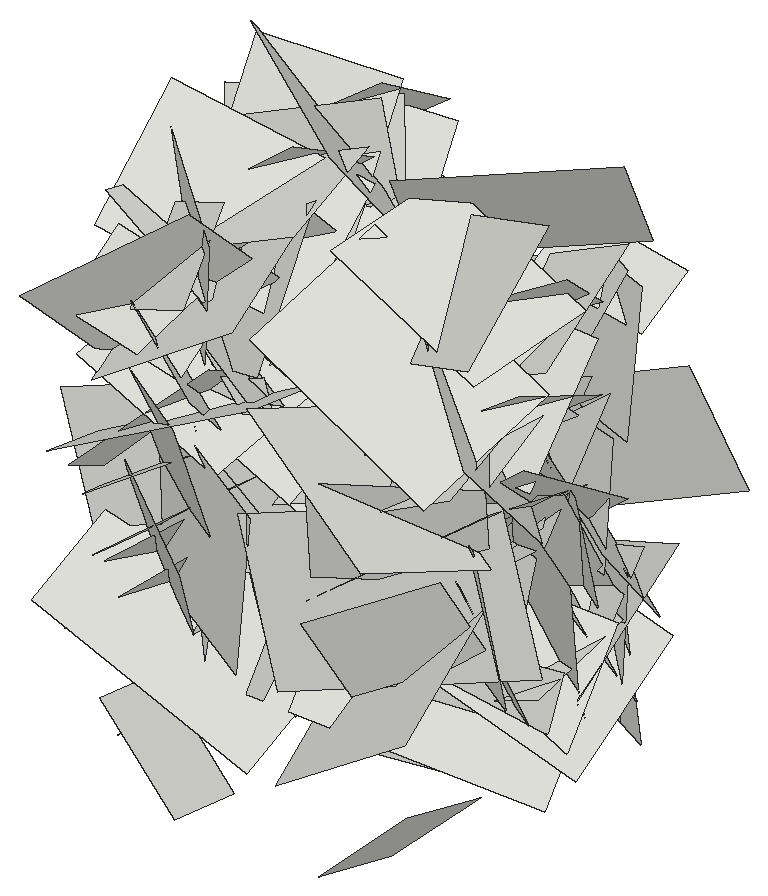
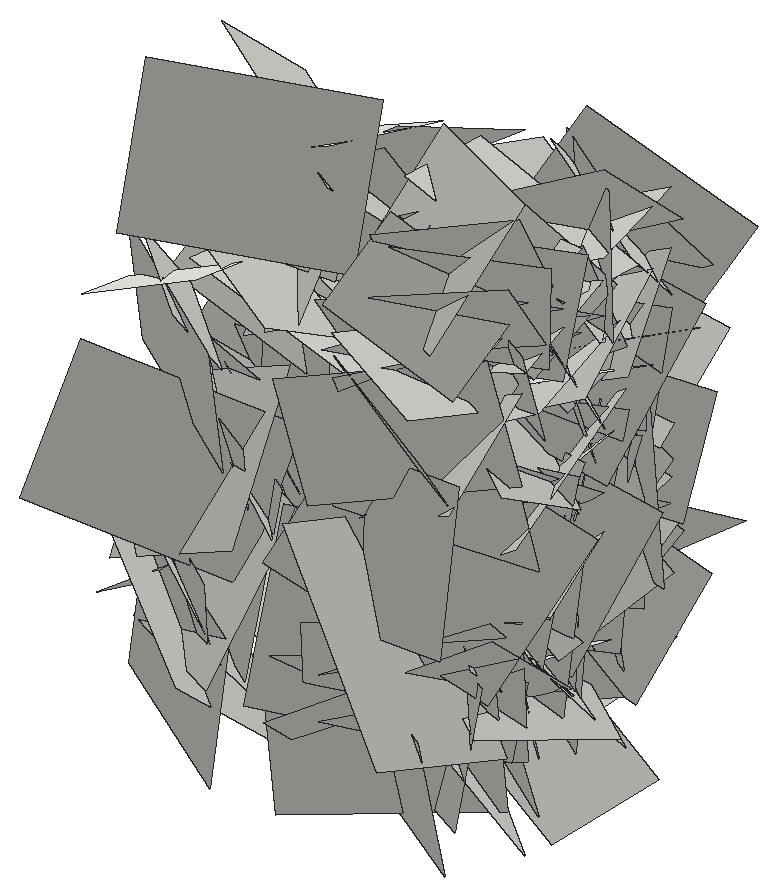
# SketchUp Ruby script. Lengths in inches.
U = 1.inch
M = Sketchup.active_model
def pt(a) = Geom::Point3d.new(a.map { |v| v * U })
def face(e, loops, mat)
  f = e.add_face(loops[0].map { |a| pt(a) })
  loops[1..].each { |l| e.add_face(l.map { |a| pt(a) }).erase! }
  f.material = f.back_material = mat if mat
  f
end
# faces: each face lists its corners as indices into pts; further lists are holes
def faces(e, pts, list, mat = nil) = list.each { |f| face(e, (f[0].is_a?(Array) ? f : [f]).map { |l| l.map { |i| pts[i] } }, mat) }
# xy, xz, yz: faces in a plane at the given z, y or x. An outline is a flat list of corners, or four numbers for a rectangle; further outlines are holes
def ring(l) = l.size == 4 ? [[l[0], l[1]], [l[2], l[1]], [l[2], l[3]], [l[0], l[3]]] : l.each_slice(2).to_a
def flat(e, list, mat, &to3) = list.each { |f| face(e, (f[0].is_a?(Array) ? f : [f]).map { |l| ring(l).map { |u, v| to3.(u, v) } }, mat) }
def xy(e, z, list, mat = nil) = flat(e, list, mat) { |x, y| [x, y, z] }
def xz(e, y, list, mat = nil) = flat(e, list, mat) { |x, z| [x, y, z] }
def yz(e, x, list, mat = nil) = flat(e, list, mat) { |y, z| [x, y, z] }
def lines(e, pts, list) = list.each { |a, b| e.add_line(pt(pts[a]), pt(pts[b])) }
# prism: a flat outline (further loops are holes) pulled along v
def prism(e, loops, v, mat = nil)
  f = face(e, loops, mat); d = Geom::Vector3d.new(v.map { |x| x * U })
  f.pushpull(f.normal.samedirection?(d) ? d.length : -d.length)
end
def box(e, o, s, mat = nil) = prism(e, [[o, [o[0] + s[0], o[1], o[2]], [o[0] + s[0], o[1] + s[1], o[2]], [o[0], o[1] + s[1], o[2]]]], [0, 0, s[2]], mat)
def at(x, y, z, deg = 0) = Geom::Transformation.translation(pt([x, y, z])) * Geom::Transformation.rotation(ORIGIN, Z_AXIS, deg.degrees)
def axes(o, x, y, z) = Geom::Transformation.new([*x, 0, *y, 0, *z, 0, *pt(o).to_a, 1])
def part(name) = M.definitions.add(name)
# library, detail: a bought-in or finely detailed component or shape, given as its bounding box
def library(name, o, s) = part(name).tap { |d| box(d.entities, o, s) }
def detail(e, o, s) = box(e.add_group.entities, o, s)
def put(e, d, t, mat = nil) = e.add_instance(d, t).tap { |i| i.material = mat if mat }
def group(e, t, mat = nil) = e.add_group.tap { |g| g.transformation = t; g.material = mat if mat }.entities
root = M.entities
c1 = part("Component\#6")
p = [[0.01,0,0],[0,3.24,4.54],[4.32,3.24,4.54],[4.33,0,0]]
faces(c1.entities,p,[[0,1,2,3]])
put(root,c1,axes([24.34,199.18,25.47],[0.11604,-0.3767,0.6399],[-0.02749,0.64448,0.38383],[0.78661,0.07809,-0.08099]))
put(root,c1,axes([24.34,201.02,32],[-0.03236,-0.79816,-0.43551],[-0.07074,-0.43262,0.79753],[0.9612,-0.0587,0.04403]))
put(root,c1,axes([28.31,202.06,39.63],[0.00244,-0.36914,-0.6705],[-0.07457,-0.66776,0.36739],[-0.80789,0.06052,-0.03594]))
put(root,c1,axes([24.34,194.18,31.13],[-0.04063,-0.16003,0.87853],[-0.02386,0.87924,0.15917],[0.94627,0.0153,0.04174]))
put(root,c1,axes([24.34,191.375,35.34],[0.1473,0.40574,0.51918],[0.07991,0.51733,-0.42447],[0.69387,-0.14571,-0.06134]))
put(root,c1,axes([28.31,192.92,34.17],[0.15147,-0.1521,1.01718],[0.1212,1.02293,0.1369],[-1.08344,0.09316,0.15752]))
put(root,c1,axes([28.31,201.02,39.48],[0.13577,0.09163,-0.9618],[0.05798,-0.96935,-0.08506],[-1.02248,-0.0428,-0.13253]))
put(root,c1,axes([28.31,193.07,33.95],[-0.05953,0.85388,-0.40475],[0.24794,-0.38029,-0.83472],[-0.97048,-0.14953,-0.18843]))
put(root,c1,axes([24.34,198.86,35.2],[-0.14047,0.16017,0.87964],[0.13868,0.88315,-0.1411],[0.93754,-0.10664,0.15267]))
put(root,c1,axes([24.34,198.41,25.5],[-0.14641,-1.02966,0.26735],[-0.10928,0.28128,1.03005],[1.12233,-0.10694,0.13517]))
put(root,c1,axes([28.31,192.38,31.46],[-0.05244,0.73173,-0.11131],[-0.01157,-0.11227,-0.73318],[-0.78447,-0.04726,0.01825]))
put(root,c1,axes([28.31,195.89,35.57],[0.03273,-0.74668,0.19464],[-0.06894,0.19158,0.74527],[-0.81502,-0.04619,-0.05522]))
put(root,c1,axes([24.34,195.33,34.42],[0.12228,0.30682,0.85432],[-0.19875,0.85067,-0.2802],[0.94146,0.13973,-0.17012]))
put(root,c1,axes([24.34,197.53,26.62],[0.11622,-0.11144,-0.6986],[0.08861,-0.69994,0.12478],[0.74462,0.10068,0.09418]))
put(root,c1,axes([28.31,194.17,31.15],[0.1572,-0.65225,0.62778],[0.00257,0.63643,0.66066],[-0.9596,-0.10514,0.10461]))
put(root,c1,axes([28.31,196.95,39.61],[0.06663,0.78722,-0.39485],[0.0883,-0.3994,-0.78302],[-0.92935,0.01849,-0.10271]))
put(root,c1,axes([24.34,195.16,37.28],[0.08536,-0.54597,-0.55526],[0.06407,-0.55215,0.55168],[0.82294,0.09962,0.01464]))
put(root,c1,axes([24.34,201.91,26.14],[-0.02369,0.31708,-0.9382],[-0.09459,-0.93526,-0.31396],[1.04548,-0.07743,-0.04967]))
put(root,c1,axes([28.31,198.57,33.25],[0.09717,0.14422,-0.89801],[0.11089,-0.89824,-0.13357],[-0.95769,-0.08937,-0.10658]))
put(root,c1,axes([24.34,200.1,34.99],[0.01875,0.74709,-0.59948],[-0.09315,-0.59579,-0.74508],[1.01106,-0.06874,-0.05753]))
put(root,c1,axes([28.31,192.15,39.48],[0.21361,0.71392,-0.72381],[0.12034,-0.74908,-0.70723],[-1.07091,0.05823,-0.22384]))
put(root,c1,axes([24.34,204.82,25.65],[-0.12938,-0.11687,-1.00907],[0.02351,-1.01639,0.11504],[1.07651,0.00815,-0.12379]))
put(root,c1,axes([28.31,197.17,21.41],[0.31691,0.51794,0.91951],[0.05422,0.94746,-0.55031],[-1.11735,0.19287,0.23409]))
put(root,c1,axes([24.34,195.4,26.27],[0.15303,-0.80886,0.21466],[-0.08059,0.20425,0.82078],[0.8834,0.15875,0.0377]))
put(root,c1,axes([24.34,195.7,29.31],[-0.12944,0.87645,-0.3909],[0.13192,-0.37627,-0.88251],[1.00866,0.16168,0.06525]))
put(root,c1,axes([28.31,199.74,34.07],[-0.11183,-0.60219,-0.2199],[0.02555,-0.22643,0.6085],[-0.67907,0.09065,0.0591]))
put(root,c1,axes([28.31,201.07,39.9375],[0.03161,0.68058,-0.41337],[0.06223,-0.41441,-0.67806],[-0.84176,-0.00508,-0.06565]))
put(root,c1,axes([24.34,195.45,23.05],[0.08121,0.42866,0.62692],[0.16296,0.6083,-0.43472],[0.78836,-0.1699,0.02528]))
put(root,c1,axes([28.31,196.5,26.6],[0.00001,0.64808,0.59207],[0.20568,0.57742,-0.63205],[-0.90746,0.13088,-0.14325]))
put(root,c1,axes([24.34,200.17,25.9],[0.12286,-0.34825,-0.84521],[-0.12526,-0.85054,0.33424],[0.96086,-0.06635,0.15165]))
put(root,c1,axes([24.34,194.92,22.54],[0.07164,-0.895,0.57486],[-0.24411,0.55005,0.88344],[1.1008,0.18023,0.15849]))
put(root,c1,axes([24.34,198.72,19.65],[-0.06387,-1.04135,0.05905],[-0.06023,0.06234,1.04135],[1.10396,-0.05685,0.06023]))
put(root,c1,axes([24.34,204.74,34.65],[0.08046,-0.48471,-0.63269],[0.12911,-0.62103,0.49039],[0.83492,0.14274,-0.01486]))
put(root,c1,axes([28.31,192.68,25.51],[-0.10584,0.56729,0.32604],[0.07365,0.33715,-0.56532],[-0.68964,-0.05105,-0.11041]))
put(root,c1,axes([24.34,194.12,36.42],[-0.16155,0.92195,-0.51802],[0.06641,-0.51458,-0.93426],[1.119,0.16364,-0.01934]))
put(root,c1,axes([28.31,197.11,20.7],[0.0234,0.20043,0.60552],[-0.11848,0.59772,-0.19378],[-0.66563,-0.09934,0.05578]))
put(root,c1,axes([24.34,192.76,27.5],[-0.21382,-0.08753,1.03604],[0.20559,1.03367,0.1251],[1.08277,-0.21355,0.18084]))
put(root,c1,axes([28.31,194.1,30.97],[0.07757,0.18705,0.69229],[-0.05179,0.69557,-0.18277],[-0.75837,-0.02837,0.08329]))
put(root,c1,axes([28.31,192.62,23.41],[0.0945,0.05137,0.75973],[-0.00531,0.76494,-0.05113],[-0.80713,0.00098,0.08928]))
put(root,c1,axes([28.31,194.0625,27.88],[0.03826,-0.32146,0.75655],[0.14724,0.74878,0.31153],[-0.85881,0.11405,0.08712]))
put(root,c1,axes([24.34,200.08,36.17],[0.04967,-0.3024,-0.77978],[0.15753,-0.76557,0.30582],[0.87244,0.15545,-0.01082]))
put(root,c1,axes([24.34,196.41,37.05],[0.02372,0.78814,-0.36288],[0.15491,-0.36124,-0.77556],[0.90659,0.0411,0.14202]))
put(root,c1,axes([24.34,206.72,25.52],[-0.07134,-1.27871,-0.42932],[-0.37284,-0.39835,1.24159],[1.38032,-0.17369,0.31318]))
put(root,c1,axes([24.34,198.67,35.61],[-0.10111,0.59855,0.78971],[0.15679,0.79307,-0.58323],[1.03859,-0.06146,0.16492]))
put(root,c1,axes([28.31,194.71,36.49],[0.01491,0.71707,-0.22931],[0.11795,-0.22881,-0.70868],[-0.78925,-0.02064,-0.11024]))
put(root,c1,axes([28.31,193.25,29.42],[0.0602,0.67546,-0.3863],[0.10598,-0.39045,-0.66802],[-0.81797,-0.00088,-0.11498]))
put(root,c1,axes([28.31,198.68,37.125],[-0.06347,0.58127,-0.24952],[0.07215,-0.24326,-0.58302],[-0.66662,-0.08167,-0.03935]))
put(root,c1,axes([24.34,195.125,35.61],[0.03117,0.92717,-0.40656],[-0.02653,-0.40594,-0.92757],[1.07281,-0.03698,-0.01113]))
put(root,c1,axes([28.31,200.57,36.04],[0.10099,0.61602,0.17436],[-0.1325,0.19079,-0.60575],[-0.66557,0.05549,0.14705]))
put(root,c1,axes([24.34,197.34,38.49],[0.22162,0.66132,-0.53694],[-0.02723,-0.54773,-0.68462],[0.90256,-0.17891,0.1112]))
put(root,c1,axes([24.34,198.8,27.02],[-0.0226,-0.2767,0.96977],[0.06915,0.96758,0.27751],[1.06674,-0.06859,0.00256]))
put(root,c1,axes([24.34,193.58,33.2],[0.1306,0.22319,-0.86205],[0.05382,-0.87061,-0.21815],[0.94237,0.01879,0.13193]))
put(root,c1,axes([24.34,197.85,24.73],[-0.35143,-0.52734,1.13432],[0.18025,1.14359,0.58135],[1.31365,-0.29799,0.22369]))
put(root,c1,axes([28.31,196.3,29.33],[0.09147,0.43894,-0.4809],[-0.05464,-0.47898,-0.44644],[-0.688,0.09639,-0.02848]))
put(root,c1,axes([28.31,192.39,25.48],[0.15082,-0.34829,0.66058],[0.01541,0.67363,0.35204],[-0.79143,-0.05326,0.13274]))
put(root,c1,axes([24.34,199.8,22.82],[-0.00598,0.07204,1.08492],[-0.02761,1.08461,-0.07215],[1.15221,0.02636,0.0039]))
put(root,c1,axes([28.31,194.26,19.42],[0.05867,-0.70774,0.13488],[0.12622,0.14241,0.69835],[-0.75321,-0.03127,0.12754]))
put(root,c1,axes([24.34,196.22,30.25],[-0.08073,-0.93811,0.99109],[-0.27356,0.98462,0.91216],[1.42044,0.13631,0.232]))
put(root,c1,axes([24.34,191.97,33.56],[0.08688,0.89449,0.25558],[0.12211,0.24484,-0.89383],[0.97851,-0.10998,0.08885]))
put(root,c1,axes([24.34,197.83,24.35],[-0.09568,0.96283,0.81475],[-0.1112,0.80827,-0.9668],[1.33234,0.1366,-0.02218]))
put(root,c1,axes([24.34,199.05,27.98],[0.08019,0.19915,0.92966],[0.13728,0.92174,-0.20799],[0.9984,-0.14274,-0.04607]))
put(root,c1,axes([24.34,202.95,33.21],[-0.17447,0.42234,-1.07867],[0.17991,-1.06896,-0.44444],[1.21466,0.21899,-0.08911]))
put(root,c1,axes([24.34,201.66,25.46],[-0.21728,-0.88431,0.94199],[0.03627,0.94972,0.89901],[1.36907,-0.16551,0.12568]))
put(root,c1,axes([24.34,195.04,27.27],[0.2131,0.57774,0.71728],[0.02179,0.73117,-0.59469],[0.97604,-0.14247,-0.14333]))
put(root,c1,axes([24.34,197.22,25.56],[0.17769,-0.12121,-0.94504],[0.07151,-0.95564,0.13453],[1.00742,0.08922,0.15714]))
put(root,c1,axes([24.34,192.77,37.47],[-0.01566,0.85002,0.74451],[0.07038,0.74394,-0.84805],[1.19569,-0.03266,0.05967]))
put(root,c1,axes([28.31,203.75,35.72],[0.12855,-0.35471,-0.52952],[0.05195,-0.53223,0.36775],[-0.67359,-0.10874,-0.07269]))
put(root,c1,axes([24.34,202.23,24.6],[-0.19755,-1.2824,-0.48224],[-0.04087,-0.48158,1.29554],[1.4517,-0.18807,-0.02915]))
put(root,c1,axes([24.34,200.11,31.93],[0.08158,0.26048,1.04137],[0.05734,1.04178,-0.26458],[1.13642,-0.07126,-0.06141]))
put(root,c1,axes([24.34,198.78,35.93],[0.06513,-0.64723,-0.92238],[0.00055,-0.92374,0.64822],[1.19442,0.03572,0.05]))
put(root,c1,axes([24.34,196.35,35.86],[0.06555,0.97369,0.5362],[0.0688,0.53295,-0.97527],[1.17625,-0.08544,0.02716]))
put(root,c1,axes([24.34,195.34,33.06],[0.01901,1.14103,-0.72029],[-0.19621,-0.71146,-1.13165],[1.41679,-0.11384,-0.14706]))
put(root,c1,axes([24.34,197.73,24.08],[0.06299,0.80841,0.87356],[-0.01823,0.87514,-0.8087],[1.26151,-0.02772,-0.0553]))
put(root,c1,axes([24.34,194.3,32.47],[-0.23408,0.14056,-1.33491],[0.22407,-1.33233,-0.17526],[1.40507,0.23589,-0.19445]))
put(root,c1,axes([24.34,196.04,25.17],[0.02819,1.07686,0.22249],[0.25409,0.21152,-1.05244],[1.13755,-0.07393,0.22957]))
put(root,c1,axes([24.34,193.85,32.27],[0.12737,1.17977,-0.33684],[-0.1012,-0.32843,-1.18439],[1.29659,-0.14153,-0.05935]))
put(root,c1,axes([24.34,198.24,37.08],[0.15669,-0.99926,-0.19378],[0.22295,-0.1616,0.99377],[1.05566,0.18244,-0.18112]))
put(root,c1,axes([24.34,197.21,31.46],[0.04455,0.58157,-0.95839],[0.2239,-0.94599,-0.56478],[1.16701,0.1593,0.14494]))
put(root,c1,axes([24.34,200.75,21.625],[0.14431,-0.01788,1.13958],[0.06693,1.14604,0.01044],[1.20625,-0.06145,-0.13692]))
put(root,c1,axes([24.34,198.29,23.22],[0.04433,-0.32511,1.32538],[-0.126,1.3201,0.32757],[1.44106,0.12543,-0.01213]))
put(root,c1,axes([24.34,196.35,30.1],[0.25467,1.00338,0.64071],[-0.12934,0.67094,-1.00496],[1.25528,-0.13443,-0.23354]))
put(root,c1,axes([24.34,199.72,26.12],[-0.08735,-0.8928,-1.02237],[0.07635,-1.02569,0.88989],[1.43674,0.00023,-0.10945]))
put(root,c1,axes([24.34,196.54,35.06],[0.17609,-1.11494,-0.45613],[-0.00034,-0.46049,1.12547],[1.27691,0.15363,0.0632]))
put(root,c1,axes([24.34,189.88,26.35],[0.12674,1.17916,0.69894],[-0.07675,0.70605,-1.17877],[1.45096,-0.06565,-0.1234]))
put(root,c1,axes([24.34,194.52,25.48],[0.11423,-0.20624,1.26777],[0.06819,1.2715,0.20138],[1.3598,-0.04643,-0.1166]))
put(root,c1,axes([24.34,193.84,30.46],[0.25587,-1.06575,0.3461],[0.15582,0.3811,1.07099],[1.17751,0.18115,-0.21693]))
put(root,c1,axes([24.34,199.97,41.09],[0.2759,0.65189,-0.94787],[0.07756,-0.97924,-0.65337],[1.21695,-0.08538,0.25653]))
put(root,c1,axes([24.34,200.57,23.13],[0.2198,-0.69796,1.13548],[-0.0671,1.14269,0.71395],[1.41122,0.16304,-0.1429]))
put(root,c1,axes([24.34,195.625,24.52],[0.22176,-0.47224,1.18941],[0.10161,1.2076,0.46259],[1.3527,-0.0133,-0.22974]))
put(root,c1,axes([24.34,193.54,33.12],[0.22081,1.30446,0.31828],[0.37279,0.25784,-1.28691],[1.3736,-0.27967,0.29809]))
put(root,c1,axes([38.11,193.54,33.12],[-0.22081,1.30446,0.31828],[-0.37279,0.25784,-1.28691],[-1.3736,-0.27967,0.29809]))
put(root,c1,axes([38.11,195.625,24.52],[-0.22176,-0.47224,1.18941],[-0.10161,1.2076,0.46259],[-1.3527,-0.0133,-0.22974]))
put(root,c1,axes([38.11,200.57,23.13],[-0.2198,-0.69796,1.13548],[0.0671,1.14269,0.71395],[-1.41122,0.16304,-0.1429]))
put(root,c1,axes([38.11,199.97,41.09],[-0.2759,0.65189,-0.94787],[-0.07756,-0.97924,-0.65337],[-1.21695,-0.08538,0.25653]))
put(root,c1,axes([38.11,193.84,30.46],[-0.25587,-1.06575,0.3461],[-0.15582,0.3811,1.07099],[-1.17751,0.18115,-0.21693]))
put(root,c1,axes([38.11,194.52,25.48],[-0.11423,-0.20624,1.26777],[-0.06819,1.2715,0.20138],[-1.3598,-0.04643,-0.1166]))
put(root,c1,axes([38.11,189.88,26.35],[-0.12674,1.17916,0.69894],[0.07675,0.70605,-1.17877],[-1.45096,-0.06565,-0.1234]))
put(root,c1,axes([38.11,196.54,35.06],[-0.17609,-1.11494,-0.45613],[0.00034,-0.46049,1.12547],[-1.27691,0.15363,0.0632]))
put(root,c1,axes([38.11,199.72,26.12],[0.08735,-0.8928,-1.02237],[-0.07635,-1.02569,0.88989],[-1.43674,0.00023,-0.10945]))
put(root,c1,axes([38.11,196.35,30.1],[-0.25467,1.00338,0.64071],[0.12934,0.67094,-1.00496],[-1.25528,-0.13443,-0.23354]))
put(root,c1,axes([38.11,198.29,23.22],[-0.04433,-0.32511,1.32538],[0.126,1.3201,0.32757],[-1.44106,0.12543,-0.01213]))
put(root,c1,axes([38.11,200.75,21.625],[-0.14431,-0.01788,1.13958],[-0.06693,1.14604,0.01044],[-1.20625,-0.06145,-0.13692]))
put(root,c1,axes([38.11,197.21,31.46],[-0.04455,0.58157,-0.95839],[-0.2239,-0.94599,-0.56478],[-1.16701,0.1593,0.14494]))
put(root,c1,axes([38.11,198.24,37.08],[-0.15669,-0.99926,-0.19378],[-0.22295,-0.1616,0.99377],[-1.05566,0.18244,-0.18112]))
put(root,c1,axes([38.11,193.85,32.27],[-0.12737,1.17977,-0.33684],[0.1012,-0.32843,-1.18439],[-1.29659,-0.14153,-0.05935]))
put(root,c1,axes([38.11,196.04,25.17],[-0.02819,1.07686,0.22249],[-0.25409,0.21152,-1.05244],[-1.13755,-0.07393,0.22957]))
put(root,c1,axes([38.11,194.3,32.47],[0.23408,0.14056,-1.33491],[-0.22407,-1.33233,-0.17526],[-1.40507,0.23589,-0.19445]))
put(root,c1,axes([38.11,197.73,24.08],[-0.06299,0.80841,0.87356],[0.01823,0.87514,-0.8087],[-1.26151,-0.02772,-0.0553]))
put(root,c1,axes([38.11,195.34,33.06],[-0.01901,1.14103,-0.72029],[0.19621,-0.71146,-1.13165],[-1.41679,-0.11384,-0.14706]))
put(root,c1,axes([38.11,196.35,35.86],[-0.06555,0.97369,0.5362],[-0.0688,0.53295,-0.97527],[-1.17625,-0.08544,0.02716]))
put(root,c1,axes([38.11,198.78,35.93],[-0.06513,-0.64723,-0.92238],[-0.00055,-0.92374,0.64822],[-1.19442,0.03572,0.05]))
put(root,c1,axes([38.11,200.11,31.93],[-0.08158,0.26048,1.04137],[-0.05734,1.04178,-0.26458],[-1.13642,-0.07126,-0.06141]))
put(root,c1,axes([38.11,202.23,24.6],[0.19755,-1.2824,-0.48224],[0.04087,-0.48158,1.29554],[-1.4517,-0.18807,-0.02915]))
put(root,c1,axes([34.14,203.75,35.72],[-0.12855,-0.35471,-0.52952],[-0.05195,-0.53223,0.36775],[0.67359,-0.10874,-0.07269]))
put(root,c1,axes([38.11,192.77,37.47],[0.01566,0.85002,0.74451],[-0.07038,0.74394,-0.84805],[-1.19569,-0.03266,0.05967]))
put(root,c1,axes([38.11,197.22,25.56],[-0.17769,-0.12121,-0.94504],[-0.07151,-0.95564,0.13453],[-1.00742,0.08922,0.15714]))
put(root,c1,axes([38.11,195.04,27.27],[-0.2131,0.57774,0.71728],[-0.02179,0.73117,-0.59469],[-0.97604,-0.14247,-0.14333]))
put(root,c1,axes([38.11,201.66,25.46],[0.21728,-0.88431,0.94199],[-0.03627,0.94972,0.89901],[-1.36907,-0.16551,0.12568]))
put(root,c1,axes([38.11,202.95,33.21],[0.17447,0.42234,-1.07867],[-0.17991,-1.06896,-0.44444],[-1.21466,0.21899,-0.08911]))
put(root,c1,axes([38.11,199.05,27.98],[-0.08019,0.19915,0.92966],[-0.13728,0.92174,-0.20799],[-0.9984,-0.14274,-0.04607]))
put(root,c1,axes([38.11,197.83,24.35],[0.09568,0.96283,0.81475],[0.1112,0.80827,-0.9668],[-1.33234,0.1366,-0.02218]))
put(root,c1,axes([38.11,191.97,33.56],[-0.08688,0.89449,0.25558],[-0.12211,0.24484,-0.89383],[-0.97851,-0.10998,0.08885]))
put(root,c1,axes([38.11,196.22,30.25],[0.08073,-0.93811,0.99109],[0.27356,0.98462,0.91216],[-1.42044,0.13631,0.232]))
put(root,c1,axes([34.14,194.26,19.42],[-0.05867,-0.70774,0.13488],[-0.12622,0.14241,0.69835],[0.75321,-0.03127,0.12754]))
put(root,c1,axes([38.11,199.8,22.82],[0.00598,0.07204,1.08492],[0.02761,1.08461,-0.07215],[-1.15221,0.02636,0.0039]))
put(root,c1,axes([34.14,192.39,25.48],[-0.15082,-0.34829,0.66058],[-0.01541,0.67363,0.35204],[0.79143,-0.05326,0.13274]))
put(root,c1,axes([34.14,196.3,29.33],[-0.09147,0.43894,-0.4809],[0.05464,-0.47898,-0.44644],[0.688,0.09639,-0.02848]))
put(root,c1,axes([38.11,197.85,24.73],[0.35143,-0.52734,1.13432],[-0.18025,1.14359,0.58135],[-1.31365,-0.29799,0.22369]))
put(root,c1,axes([38.11,193.58,33.2],[-0.1306,0.22319,-0.86205],[-0.05382,-0.87061,-0.21815],[-0.94237,0.01879,0.13193]))
put(root,c1,axes([38.11,198.8,27.02],[0.0226,-0.2767,0.96977],[-0.06915,0.96758,0.27751],[-1.06674,-0.06859,0.00256]))
put(root,c1,axes([38.11,197.34,38.49],[-0.22162,0.66132,-0.53694],[0.02723,-0.54773,-0.68462],[-0.90256,-0.17891,0.1112]))
put(root,c1,axes([34.14,200.57,36.04],[-0.10099,0.61602,0.17436],[0.1325,0.19079,-0.60575],[0.66557,0.05549,0.14705]))
put(root,c1,axes([38.11,195.125,35.61],[-0.03117,0.92717,-0.40656],[0.02653,-0.40594,-0.92757],[-1.07281,-0.03698,-0.01113]))
